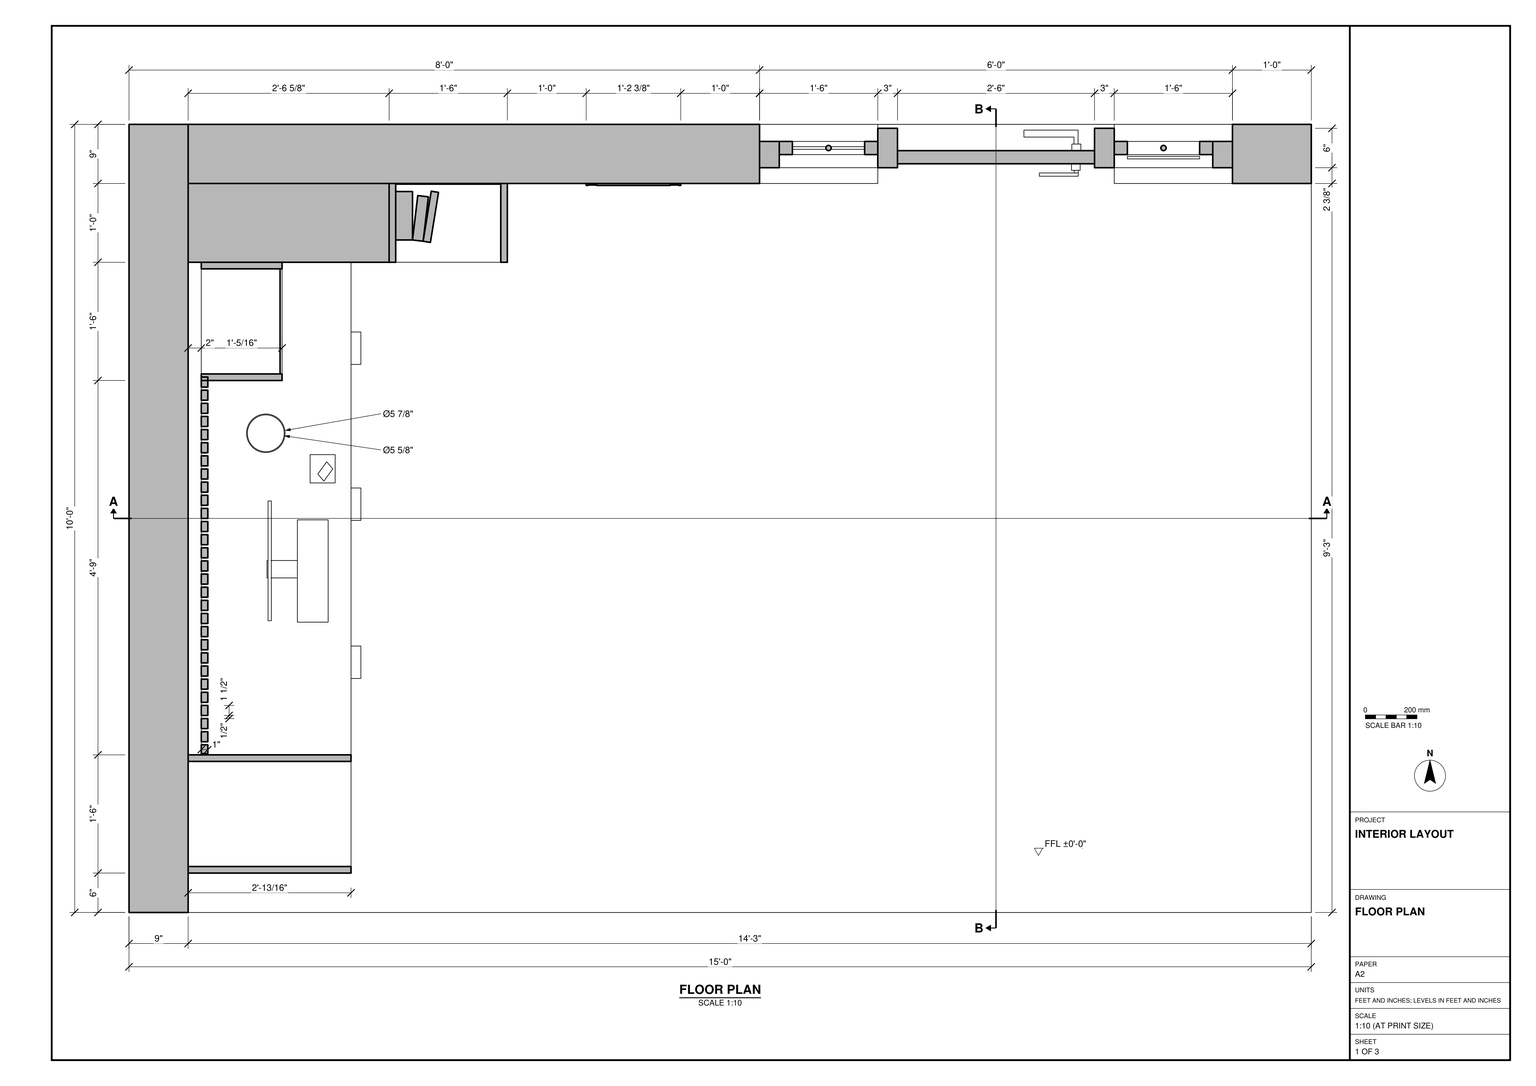
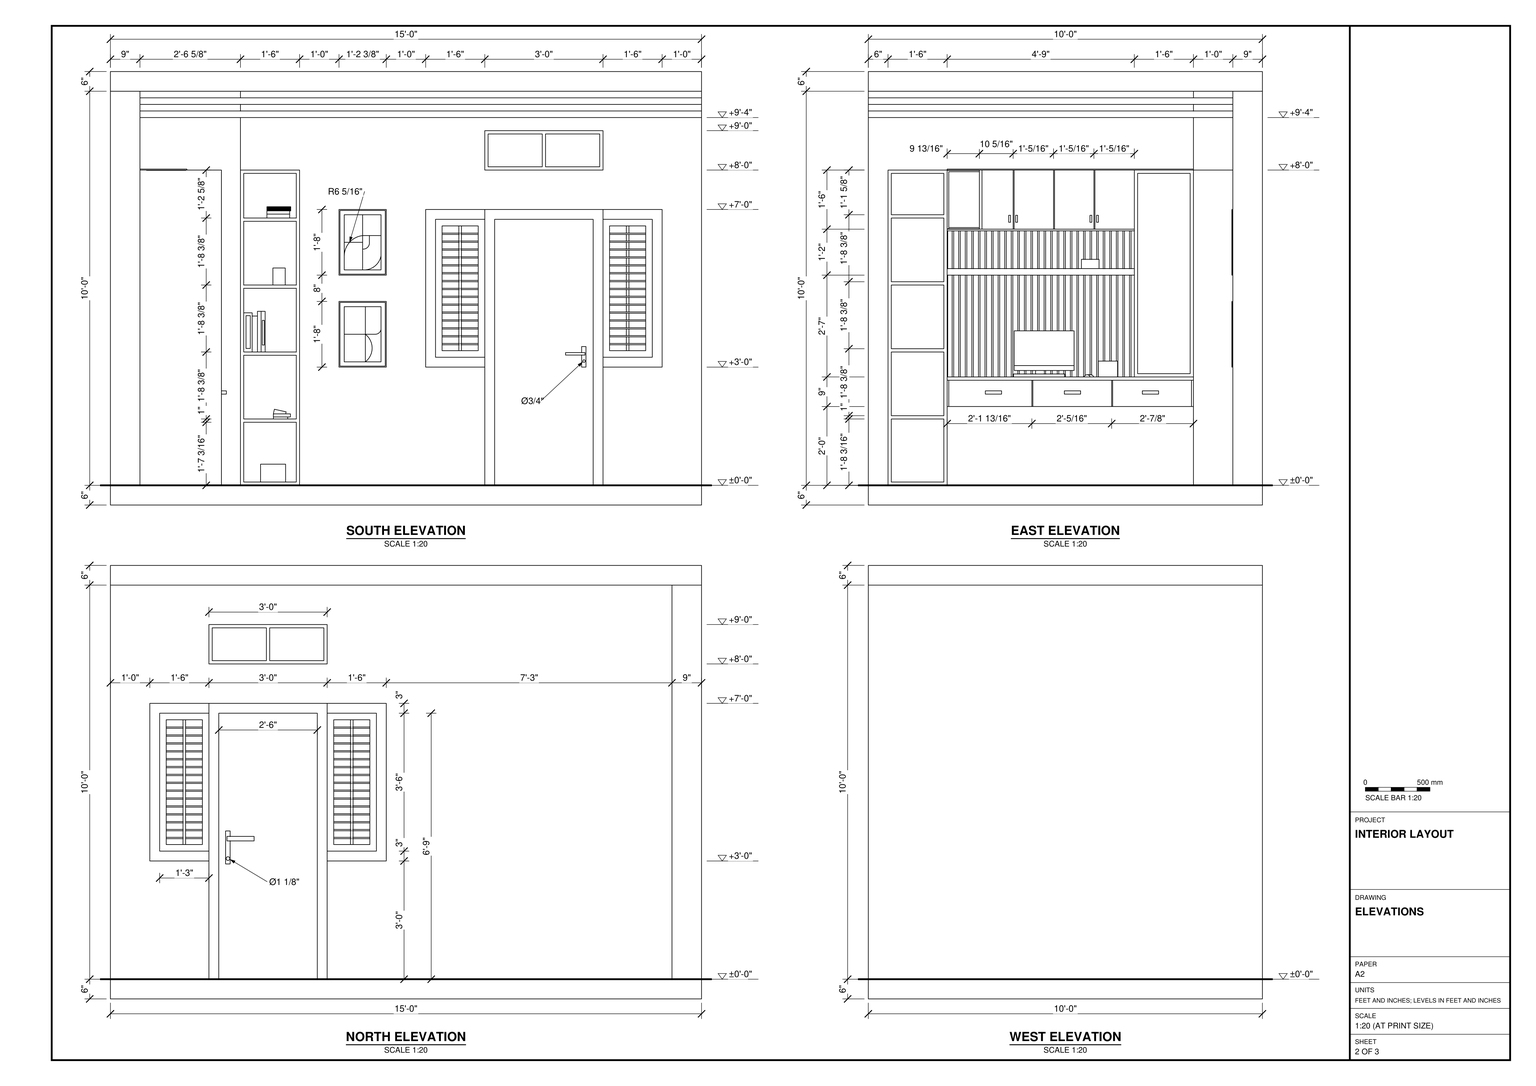
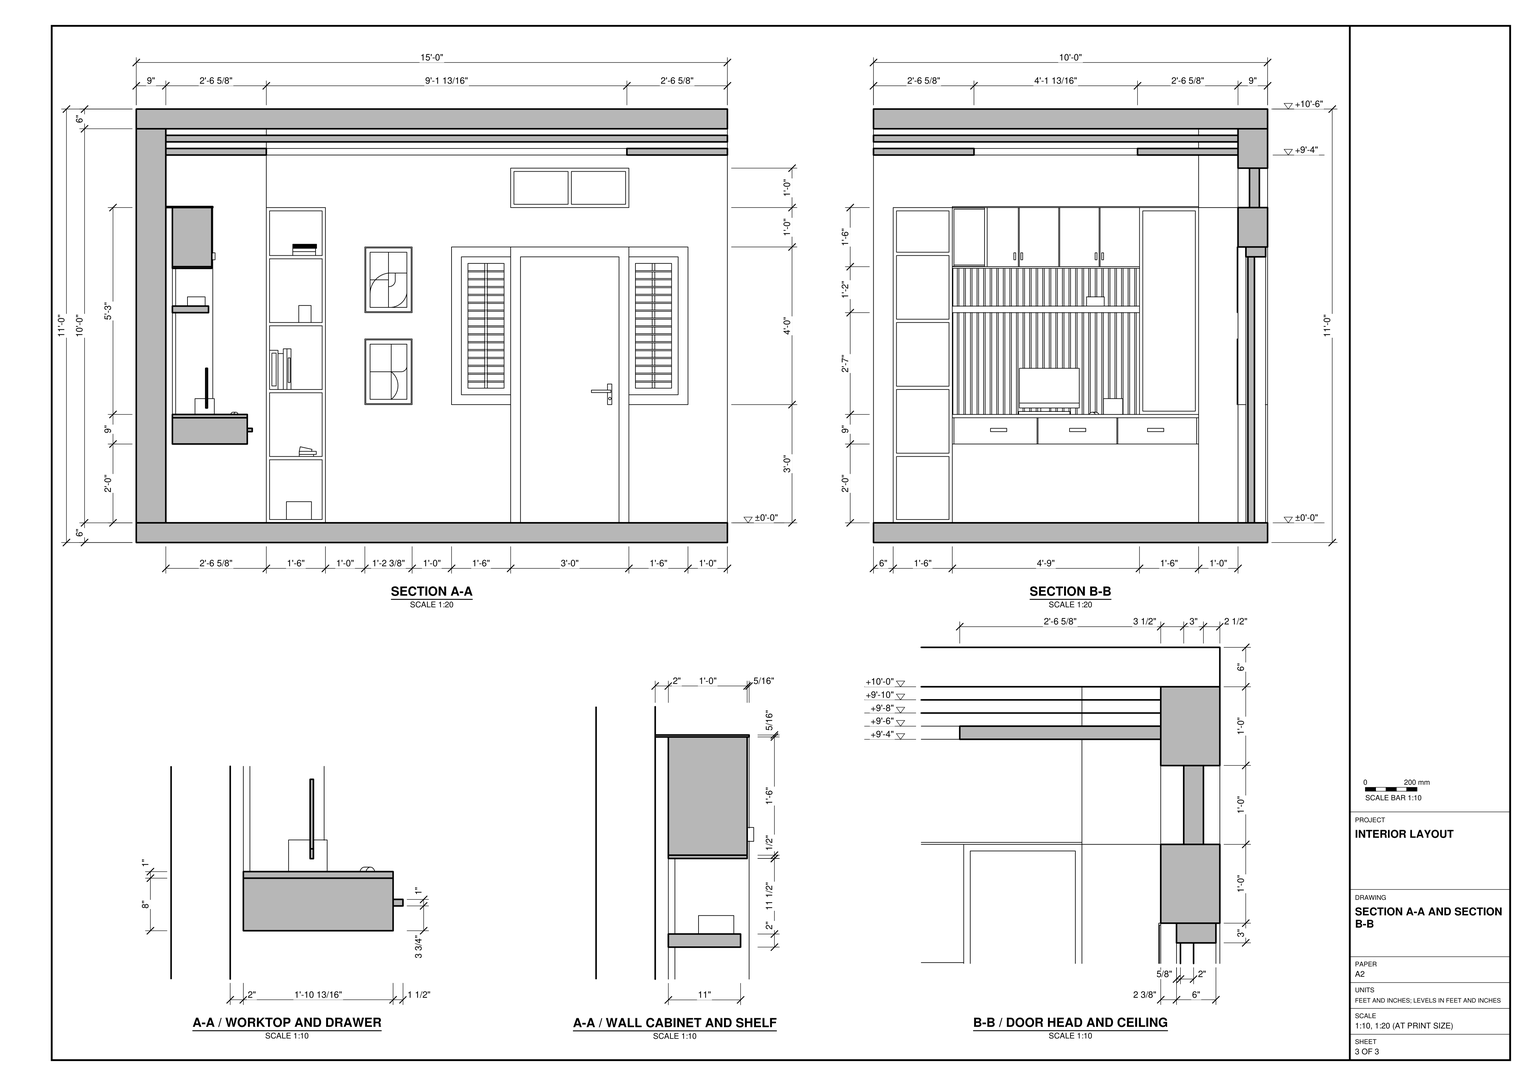
Build the interior in SketchUp from task_files/diagram_01.pdf. Work in feet and inches. Use the finished floor at ±0'-0" as the single storey datum. The model is 15'-0" along the entrance wall, 10'-0" along the workstation wall and 11'-0" high from the underside of the floor slab to the top of the roof slab.

Model the two adjoining 9" walls shown in plan, leaving the other two sides open. Include the floor and roof slabs and follow the door-head section for the stepped ceiling beneath the roof slab. Set the door toward the east end of the north wall, between two narrow louvred windows, with a separate two-pane window above it.

Fit out the west wall with the suspended worktop and drawers, vertical slatted backing, shelf, overhead cupboards and storage at each end. Use the enlarged sections to set the depths of the worktop, shelf and cupboards. Include the open shelving on the adjoining north wall, the monitor on the worktop and the pair of framed pictures between the shelving and the doorway. Decor and loose items may be any suitable library components.

Keep the walls, slabs and each furniture or joinery piece in separate groups or components, and use components for repeated parts. Save one SketchUp model as output_files/room_with_a_fitted_workstation_and_flanked_doorway.skp.

# SketchUp Ruby script. Lengths in inches.
U = 1.inch
M = Sketchup.active_model
def pt(a) = Geom::Point3d.new(a.map { |v| v * U })
def face(e, loops, mat)
  f = e.add_face(loops[0].map { |a| pt(a) })
  loops[1..].each { |l| e.add_face(l.map { |a| pt(a) }).erase! }
  f.material = f.back_material = mat if mat
  f
end
# faces: each face lists its corners as indices into pts; further lists are holes
def faces(e, pts, list, mat = nil) = list.each { |f| face(e, (f[0].is_a?(Array) ? f : [f]).map { |l| l.map { |i| pts[i] } }, mat) }
# xy, xz, yz: faces in a plane at the given z, y or x. An outline is a flat list of corners, or four numbers for a rectangle; further outlines are holes
def ring(l) = l.size == 4 ? [[l[0], l[1]], [l[2], l[1]], [l[2], l[3]], [l[0], l[3]]] : l.each_slice(2).to_a
def flat(e, list, mat, &to3) = list.each { |f| face(e, (f[0].is_a?(Array) ? f : [f]).map { |l| ring(l).map { |u, v| to3.(u, v) } }, mat) }
def xy(e, z, list, mat = nil) = flat(e, list, mat) { |x, y| [x, y, z] }
def xz(e, y, list, mat = nil) = flat(e, list, mat) { |x, z| [x, y, z] }
def yz(e, x, list, mat = nil) = flat(e, list, mat) { |y, z| [x, y, z] }
def lines(e, pts, list) = list.each { |a, b| e.add_line(pt(pts[a]), pt(pts[b])) }
# prism: a flat outline (further loops are holes) pulled along v
def prism(e, loops, v, mat = nil)
  f = face(e, loops, mat); d = Geom::Vector3d.new(v.map { |x| x * U })
  f.pushpull(f.normal.samedirection?(d) ? d.length : -d.length)
end
def box(e, o, s, mat = nil) = prism(e, [[o, [o[0] + s[0], o[1], o[2]], [o[0] + s[0], o[1] + s[1], o[2]], [o[0], o[1] + s[1], o[2]]]], [0, 0, s[2]], mat)
def at(x, y, z, deg = 0) = Geom::Transformation.translation(pt([x, y, z])) * Geom::Transformation.rotation(ORIGIN, Z_AXIS, deg.degrees)
def axes(o, x, y, z) = Geom::Transformation.new([*x, 0, *y, 0, *z, 0, *pt(o).to_a, 1])
def part(name) = M.definitions.add(name)
# library, detail: a bought-in or finely detailed component or shape, given as its bounding box
def library(name, o, s) = part(name).tap { |d| box(d.entities, o, s) }
def detail(e, o, s) = box(e.add_group.entities, o, s)
def put(e, d, t, mat = nil) = e.add_instance(d, t).tap { |i| i.material = mat if mat }
def group(e, t, mat = nil) = e.add_group.tap { |g| g.transformation = t; g.material = mat if mat }.entities
root = M.entities
M.materials.add("[0014_DarkSalmon]").color = [233, 150, 122]
M.materials.add("[0034_Wheat]").color = [245, 222, 179]
M.materials.add("[0040_Peru]").color = [205, 133, 63]
M.materials.add("[0050_LemonChiffon]").color = [255, 250, 205]
M.materials.add("[0052_FloralWhite]").color = [255, 250, 240]
M.materials.add("[0137_Black]").color = [0, 0, 0]
M.materials.add("[Color A08]").color = [102, 0, 0]
M.materials.add("[Color D02]").color = [214, 192, 128]
M.materials.add("[Color D07]").color = [153, 114, 0]
M.materials.add("[Color E01]").color = [242, 242, 193]
M.materials.add("[Color E01]1").color = [255, 255, 204]
M.materials.add("[Color L16]").color = [102, 0, 51]
M.materials.add("[Color M00]").color = [255, 255, 255]
M.materials.add("[Color M06]").color = [86, 86, 86]
M.materials.add("[Color M07]").color = [58, 58, 58]
M.materials.add("[Color M09]").color = [0, 0, 0]
M.materials.add("[Metal Aluminum Anodized]").color = [202, 209, 219]
M.materials.add("[Translucent Glass Blue]").color = [107, 160, 255]
M.materials.add("[Translucent Glass Gray]").color = [128, 128, 128]
M.materials.add("[Vegetation Juniper]").color = [99, 128, 70]
M.materials.add("[Wood Veneer 01]").color = [112, 65, 34]
M.materials.add("[Wood Veneer 01]1").color = [84, 49, 25]
c1 = part("Group\#11")
prism(c1.entities,[[[0,0.27,0.01],[0,0.22,0],[0,0.17,0],[0,0.12,0.02],[0,0.07,0.04],[0,0.04,0.08],[0,0.01,0.13],[0,0,0.18],[0,0,0.23],[0,0.02,0.28],[0,0.04,0.33],[0,0.08,0.36],[0,0.13,0.39],[0,0.18,0.4],[0,0.23,0.4],[0,0.28,0.38],[0,0.33,0.35],[0,0.36,0.32],[0,0.39,0.27],[0,0.4,0.22],[0,0.4,0.17],[0,0.38,0.12],[0,0.35,0.07],[0,0.32,0.04]]],[11,0,0])
c2 = part("Group\#9")
xy(c2.entities,0,[[0,0,15,2]])
xy(c2.entities,2,[[[2,0,13,2],[7.5,0.6,7.4,0.61,7.3,0.65,7.22,0.72,7.15,0.8,7.11,0.9,7.1,1,7.11,1.1,7.15,1.2,7.22,1.28,7.3,1.35,7.4,1.39,7.5,1.4,7.6,1.39,7.7,1.35,7.78,1.28,7.85,1.2,7.89,1.1,7.9,1,7.89,0.9,7.85,0.8,7.78,0.72,7.7,0.65,7.6,0.61]]])
xy(c2.entities,40,[[[2,0,13,2],[7.5,0.6,7.6,0.61,7.7,0.65,7.78,0.72,7.85,0.8,7.89,0.9,7.9,1,7.89,1.1,7.85,1.2,7.78,1.28,7.7,1.35,7.6,1.39,7.5,1.4,7.4,1.39,7.3,1.35,7.22,1.28,7.15,1.2,7.11,1.1,7.1,1,7.11,0.9,7.15,0.8,7.22,0.72,7.3,0.65,7.4,0.61]]])
xy(c2.entities,42,[[0,0,15,2]])
xz(c2.entities,0,[[[0,0,15,42],[2,2,13,40]]])
xz(c2.entities,2,[[[0,0,15,42],[2,2,13,40]]])
yz(c2.entities,0,[[0,0,2,42]])
yz(c2.entities,2,[[0,2,2,40]])
yz(c2.entities,13,[[0,2,2,40]])
yz(c2.entities,15,[[0,0,2,42]])
p = [[7.3,0.65,2],[7.4,0.61,2],[7.4,0.61,40],[7.3,0.65,40],[7.5,0.6,2],[7.5,0.6,40],
  [7.6,0.61,2],[7.6,0.61,40],[7.7,0.65,2],[7.7,0.65,40],[7.15,0.8,2],[7.22,0.72,2],
  [7.22,0.72,40],[7.15,0.8,40],[7.78,0.72,2],[7.78,0.72,40],[7.85,0.8,2],[7.85,0.8,40],
  [7.11,0.9,2],[7.11,0.9,40],[7.89,0.9,2],[7.89,0.9,40],[7.1,1,2],[7.1,1,40],
  [7.9,1,2],[7.9,1,40],[7.11,1.1,2],[7.11,1.1,40],[7.89,1.1,2],[7.89,1.1,40],
  [7.15,1.2,2],[7.15,1.2,40],[7.85,1.2,2],[7.85,1.2,40],[7.22,1.28,2],[7.22,1.28,40],
  [7.78,1.28,2],[7.78,1.28,40],[7.3,1.35,2],[7.3,1.35,40],[7.4,1.39,2],[7.4,1.39,40],
  [7.7,1.35,2],[7.6,1.39,2],[7.6,1.39,40],[7.7,1.35,40],[7.5,1.4,2],[7.5,1.4,40]]
faces(c2.entities,p,[[0,1,2,3],[1,4,5,2],[4,6,7,5],[6,8,9,7],[10,11,12,13],[11,0,3,12],[8,14,15,9],[14,16,17,15],
  [18,10,13,19],[16,20,21,17],[22,18,19,23],[20,24,25,21],[26,22,23,27],[24,28,29,25],[30,26,27,31],[28,32,33,29],
  [34,30,31,35],[32,36,37,33],[38,34,35,39],[40,38,39,41],[42,43,44,45],[36,42,45,37],[46,40,41,47],[43,46,47,44]])
c3 = part("Group\#28")
box(c3.entities,[0,0,0],[1,1.53,44.5])
c4 = part("Group\#30")
box(c4.entities,[0,0,0],[1,0.5625,2.125])
c5 = part("Group\#31")
box(c5.entities,[0,0,0],[1.5,4.9375,1])
c6 = library("Group\#43",[0,0,0],[171,111,2])
c7 = library("Group\#45",[0,0,0],[7.625,7.62,5.4375])
c8 = library("Group\#50",[0,0,0],[5.875,5.87,4.8125])
box(root,[40.6,110.9,7],[16,0.1,94],"[Color E01]")
xz(root,114.5,[[115,103,131.5,113],[132.5,103,149,113]],"[Translucent Glass Blue]")
yz(root,23,[[82,40,98,101],[24.5,84.5,33.8125,101.5]],"[Translucent Glass Gray]")
# 5 loose lines left out
g1 = group(root,at(9,111,6),"[0050_LemonChiffon]")
prism(g1,[[[105,9,0],[0,9,0],[0,9,120],[171,9,120],[171,9,0],[141,9,0],[141,9,36],[159,9,36],[159,9,84],[141,9,84],[105,9,84],[87,9,84],[87,9,36],[105,9,36]],[[105,9,108],[105,9,96],[141,9,96],[141,9,108]]],[0,-9,0])
g2 = group(root,at(96,112.1,6),"[Wood Veneer 01]")
g3 = group(g2,at(42.59,0,36),"[Metal Aluminum Anodized]")
box(g3,[0,0,3.67],[5.92,0.5,0.75])
g4 = group(g3,at(4.9,0.5,0))
xy(g4,0,[[0,0.4,1.32,1.4]])
xy(g4,3.86,[[0.41,0,1.02,0.4]])
xy(g4,4.42,[[0.41,0,1.02,0.4]])
xy(g4,6.26,[[0,0.4,1.32,1.4]])
xz(g4,0,[[0.41,3.86,1.02,4.42]])
xz(g4,0.4,[[[0,0,1.32,6.26],[0.72,1.47,0.625,1.49,0.53,1.52,0.46,1.58,0.4,1.66,0.36,1.75,0.35,1.85,0.36,1.94,0.4,2.04,0.46,2.11,0.53,2.17,0.625,2.21,0.72,2.22,0.82,2.21,0.91,2.17,0.99,2.11,1.05,2.04,1.08,1.94,1.1,1.85,1.08,1.75,1.05,1.66,0.99,1.58,0.91,1.52,0.82,1.49],[0.41,3.86,1.02,4.42]]])
xz(g4,1.4,[[0,0,1.32,6.26]])
xz(g4,1.84,[[0.72,1.47,0.82,1.49,0.91,1.52,0.99,1.58,1.05,1.66,1.08,1.75,1.1,1.85,1.08,1.94,1.05,2.04,0.99,2.11,0.91,2.17,0.82,2.21,0.72,2.22,0.625,2.21,0.53,2.17,0.46,2.11,0.4,2.04,0.36,1.94,0.35,1.85,0.36,1.75,0.4,1.66,0.46,1.58,0.53,1.52,0.625,1.49]])
yz(g4,0,[[0.4,0,1.4,6.26]])
yz(g4,0.41,[[0,3.86,0.4,4.42]])
yz(g4,1.02,[[0,3.86,0.4,4.42]])
yz(g4,1.32,[[0.4,0,1.4,6.26]])
p = [[0.46,0.4,1.58],[0.53,0.4,1.52],[0.53,1.84,1.52],[0.46,1.84,1.58],[0.625,0.4,1.49],[0.625,1.84,1.49],
  [0.72,0.4,1.47],[0.72,1.84,1.47],[0.82,0.4,1.49],[0.82,1.84,1.49],[0.91,0.4,1.52],[0.91,1.84,1.52],
  [0.99,0.4,1.58],[0.99,1.84,1.58],[0.4,0.4,1.66],[0.4,1.84,1.66],[1.05,0.4,1.66],[1.05,1.84,1.66],
  [0.36,0.4,1.75],[0.36,1.84,1.75],[1.08,0.4,1.75],[1.08,1.84,1.75],[0.35,0.4,1.85],[0.35,1.84,1.85],
  [0.36,0.4,1.94],[0.36,1.84,1.94],[1.1,0.4,1.85],[1.08,0.4,1.94],[1.08,1.84,1.94],[1.1,1.84,1.85],
  [0.4,0.4,2.04],[0.4,1.84,2.04],[1.05,0.4,2.04],[1.05,1.84,2.04],[0.46,0.4,2.11],[0.46,1.84,2.11],
  [0.99,0.4,2.11],[0.99,1.84,2.11],[0.53,0.4,2.17],[0.53,1.84,2.17],[0.91,0.4,2.17],[0.91,1.84,2.17],
  [0.625,0.4,2.21],[0.625,1.84,2.21],[0.72,0.4,2.22],[0.72,1.84,2.22],[0.82,0.4,2.21],[0.82,1.84,2.21]]
faces(g4,p,[[0,1,2,3],[1,4,5,2],[4,6,7,5],[6,8,9,7],[8,10,11,9],[10,12,13,11],[14,0,3,15],[12,16,17,13],
  [18,14,15,19],[16,20,21,17],[22,18,19,23],[24,22,23,25],[26,27,28,29],[20,26,29,21],[30,24,25,31],[27,32,33,28],
  [34,30,31,35],[32,36,37,33],[38,34,35,39],[36,40,41,37],[42,38,39,43],[44,42,43,45],[46,44,45,47],[40,46,47,41]])
g5 = group(g2,at(18,1.3,0))
prism(g5,[[[36,6,0],[33,6,0],[33,6,81],[3,6,81],[3,6,0],[0,6,0],[0,6,84],[36,6,84]]],[0,-6,0])
g6 = group(g2,at(54,1.3,36))
prism(g6,[[[15,4,45],[0,4,45],[0,4,48],[18,4,48],[18,4,0],[0,4,0],[0,4,3],[15,4,3]]],[0,-4,0])
# 1 loose lines left out
g7 = group(g2,at(0,1.3,36))
prism(g7,[[[18,4,48],[18,4,45],[3,4,45],[3,4,3],[18,4,3],[18,4,0],[0,4,0],[0,4,48]]],[0,-4,0])
# 1 loose lines left out
g8 = group(g2,at(21,1.9,0))
box(g8,[0,0,0],[30,2,81])
g9 = group(g2,at(54,1.84,39))
put(g9,c1,at(2,0.8,13.4))
put(g9,c1,at(2,0.8,3.8))
put(g9,c1,at(2,0.8,8.6))
put(g9,c1,at(2,0.8,20.6))
put(g9,c1,at(2,0.8,11))
put(g9,c1,at(2,0.8,15.8))
put(g9,c1,at(2,0.8,25.4))
put(g9,c1,at(2,0.8,23))
put(g9,c2,at(0,1.46,0))
put(g9,c1,at(2,0.8,18.2))
put(g9,c1,at(2,0.8,6.2))
put(g9,c1,at(2,0.8,37.4))
put(g9,c1,at(2,0.8,32.6))
put(g9,c1,at(2,0.8,35))
put(g9,c1,at(2,0.8,30.2))
put(g9,c1,at(2,0.8,27.8))
g10 = group(g2,at(3,3.3,39))
put(g10,c1,at(2,0.8,13.4))
put(g10,c1,at(2,0.8,3.8))
put(g10,c1,at(2,0.8,8.6))
put(g10,c1,at(2,0.8,20.6))
put(g10,c1,at(2,0.8,11))
put(g10,c1,at(2,0.8,15.8))
put(g10,c1,at(2,0.8,25.4))
put(g10,c1,at(2,0.8,23))
put(g10,c2,at(0,0,0))
put(g10,c1,at(2,0.8,18.2))
put(g10,c1,at(2,0.8,6.2))
put(g10,c1,at(2,0.8,37.4))
put(g10,c1,at(2,0.8,32.6))
put(g10,c1,at(2,0.8,35))
put(g10,c1,at(2,0.8,30.2))
put(g10,c1,at(2,0.8,27.8))
g11 = group(root,at(114,115.5,102))
prism(g11,[[[0,-1,12],[0,-1,0],[36,-1,0],[36,-1,12]],[[17.5,-1,11],[17.5,-1,1],[1,-1,1],[1,-1,11]],[[18.5,-1,11],[35,-1,11],[35,-1,1],[18.5,-1,1]]],[0,3,0])
g12 = group(root,at(0,0,6),"[0050_LemonChiffon]")
box(g12,[0,0,0],[9,120,120])
g13 = group(root,at(9,99,6),"[0050_LemonChiffon]")
xy(g13,0,[[0,0,30.6,12]])
xy(g13,120,[[0,0,30.6,12]])
xz(g13,0,[[0,0,30.6,112],[0,112,30.6,120]])
xz(g13,12,[[0,0,30.6,120]])
yz(g13,0,[[0,0,12,120]])
yz(g13,30.6,[[0,0,12,112],[0,112,12,120]])
g14 = group(root,at(0,0,0))
box(g14,[0,0,0],[180,120,6])
g15 = group(root,at(9,24,30))
g16 = group(g15,at(2,57,9),"[Wood Veneer 01]1")
xy(g16,0,[[0,0,12.3,18]])
xy(g16,1,[[0,1,12.3,17]])
xy(g16,62,[[0,1,12.3,17]])
xy(g16,63,[[0,0,12.3,18]])
xz(g16,0,[[0,0,12.3,63]])
xz(g16,1,[[0,1,12.3,62]])
xz(g16,17,[[0,1,12.3,62]])
xz(g16,18,[[0,0,12.3,63]])
yz(g16,0,[[[0,0,18,63],[1,1,17,62]]])
yz(g16,12.3,[[[0,0,18,63],[1,1,17,62]]],"[Color M00]")
g17 = group(g15,at(2,0,8),"[Wood Veneer 01]1")
box(g17,[0,0,0],[22.8,75,1])
g18 = group(g15,at(2,0,54))
xy(g18,0,[[0,0,12,9.8125],[0,9.8125,12,10.61],[0,10.61,12,20.1],[0,20.1,11.7,20.4],[0,20.4,12,32.4],
  [0,32.4,12,32.7],[0,32.7,12,44.7],[0,44.7,11.7,45],[0,45,12,57]],"[Color M00]")
xy(g18,17.9,[[0,0,12,9.8125]],"[Color M00]")
xy(g18,18,[[0,9.8125,12,10.61],[0,10.61,12,20.1],[0,20.1,11.7,20.4],[0,20.4,12,32.4],[0,32.4,12,32.7],
  [0,32.7,12,44.7],[0,44.7,11.7,45],[0,45,12,57]],"[Color M00]")
xz(g18,0,[[0,0,12,17.9]],"[Color M00]")
xz(g18,9.8125,[[0,0,12,17.9],[0,17.9,12,18]],"[Color M00]")
xz(g18,10.61,[[0,0,12,18]],"[Color M00]")
xz(g18,20.1,[[0,0,11.7,18],[11.7,0,12,18]],"[Color M00]")
xz(g18,20.4,[[0,0,11.7,18],[11.7,0,12,18]],"[Color M00]")
xz(g18,32.4,[[0,0,12,18]],"[Color M00]")
xz(g18,32.7,[[0,0,12,18]],"[Color M00]")
xz(g18,44.7,[[0,0,11.7,18],[11.7,0,12,18]],"[Color M00]")
xz(g18,45,[[0,0,11.7,18],[11.7,0,12,18]],"[Color M00]")
xz(g18,57,[[0,0,12,18]],"[Color M00]")
yz(g18,0,[[9.8125,0,10.61,18],[10.61,0,20.1,18],[20.1,0,20.4,18],[20.4,0,32.4,18],[32.4,0,32.7,18],
  [32.7,0,44.7,18],[44.7,0,45,18],[45,0,57,18],[0,17.9,9.8125,18]],"[Color M00]")
yz(g18,11.7,[[20.1,0,20.4,18],[44.7,0,45,18]],"[Color M00]")
yz(g18,12,[[0,0,9.8125,0,9.8125,0.5,0.5,0.5,0.5,17.5,9.8125,17.5,9.8125,17.9,0,17.9],[9.8125,0,10.61,18],[10.61,0,20.1,18],[20.4,0,32.4,18],[32.4,0,32.7,18],
  [32.7,0,44.7,18],[45,0,57,18]],"[Color M00]")
g19 = group(g15,at(2,-1,40),"[Wood Veneer 01]1")
box(g19,[0,1,0],[11,57,2])
g20 = group(g15,at(2,0,0))
xy(g20,0,[[0,0,22.8,0.5],[0,0.5,22.8,25.8],[0,25.8,22.5,26.1],[0,26.1,22.8,50.1],[0,50.1,22.5,50.4],
  [0,50.4,22.8,74.4],[0,74.4,22.8,75]])
xy(g20,8,[[0,0,22.8,0.5],[0,0.5,22.8,25.8],[0,25.8,22.5,26.1],[22.5,25.8,22.8,26.1],[0,26.1,22.8,50.1],
  [0,50.1,22.5,50.4],[22.5,50.1,22.8,50.4],[0,50.4,22.8,74.4],[0,74.4,22.8,75]])
xz(g20,0,[[0,0,22.8,8]])
xz(g20,0.5,[[0,0,22.8,8]])
xz(g20,25.8,[[0,0,22.5,8],[22.5,0,22.8,8]])
xz(g20,26.1,[[0,0,22.5,8],[22.5,0,22.8,8]])
xz(g20,50.1,[[0,0,22.5,8],[22.5,0,22.8,8]])
xz(g20,50.4,[[0,0,22.5,8],[22.5,0,22.8,8]])
xz(g20,74.4,[[0,0,22.8,8]])
xz(g20,75,[[0,0,22.8,8]])
yz(g20,0,[[0,0,0.5,8],[0.5,0,25.8,8],[25.8,0,26.1,8],[26.1,0,50.1,8],[50.1,0,50.4,8],
  [50.4,0,74.4,8],[74.4,0,75,8]])
yz(g20,22.5,[[25.8,0,26.1,8],[50.1,0,50.4,8]])
yz(g20,22.8,[[0,0,0.5,8],[0.5,0,25.8,8],[26.1,0,50.1,8],[50.4,0,74.4,8],[74.4,0,75,8]])
g21 = group(root,at(39.6,99,6),"[Wood Veneer 01]1")
prism(g21,[[[0,12,0],[0,12,96],[18,12,96],[18,12,0]],[[1,12,61],[17,12,61],[17,12,80.4],[1,12,80.4]],[[1,12,40.6],[17,12,40.6],[17,12,60],[1,12,60]],[[1,12,39.6],[1,12,20.2],[17,12,20.2],[17,12,39.6]],[[17,12,19.2],[1,12,19.2],[1,12,1],[17,12,1]],[[1,12,95],[1,12,81.4],[17,12,81.4],[17,12,95]]],[0,-12,0])
g22 = group(root,at(11,24,83.5),"[Wood Veneer 01]1")
box(g22,[0,0,0],[12,57,0.5])
g23 = group(root,at(11,24,39),"[Color D02]")
put(g23,c3,at(0,4,0))
g24 = group(g23,at(0,0,0))
box(g24,[0,0.1875,0],[1,1.34,44.5])
put(g23,c3,at(0,2,0))
put(g23,c3,at(0,6,0))
put(g23,c3,at(0,56,0))
put(g23,c3,at(0,46,0))
put(g23,c3,at(0,44,0))
put(g23,c3,at(0,50,0))
put(g23,c3,at(0,54,0))
put(g23,c3,at(0,52,0))
put(g23,c3,at(0,48,0))
put(g23,c3,at(0,20,0))
put(g23,c3,at(0,34,0))
put(g23,c3,at(0,38,0))
put(g23,c3,at(0,40,0))
put(g23,c3,at(0,36,0))
put(g23,c3,at(0,18,0))
put(g23,c3,at(0,8,0))
put(g23,c3,at(0,14,0))
put(g23,c3,at(0,22,0))
put(g23,c3,at(0,26,0))
put(g23,c3,at(0,30,0))
put(g23,c3,at(0,12,0))
put(g23,c3,at(0,10,0))
put(g23,c3,at(0,24,0))
put(g23,c3,at(0,28,0))
put(g23,c3,at(0,16,0))
put(g23,c3,at(0,32,0))
put(g23,c3,at(0,42,0))
g25 = group(root,at(9,24,102),"[Wood Veneer 01]1")
box(g25,[0,0,0],[14.3,75,0.3])
put(root,c4,at(23,69.49,86.1),"[Wood Veneer 01]1")
put(root,c4,at(23,67.49,86.1),"[Wood Veneer 01]1")
put(root,c4,at(23,44.86,86.1),"[Wood Veneer 01]1")
put(root,c4,at(23,42.74,86.1),"[Wood Veneer 01]1")
put(root,c5,at(33.8,35.63,33.77),"[Wood Veneer 01]1")
put(root,c5,at(33.8,59.7,33.77),"[Wood Veneer 01]1")
put(root,c5,at(33.8,83.45,33.77),"[Wood Veneer 01]1")
g26 = group(root,at(21,44.2,39))
box(g26,[4.625,0,0],[4.6875,15.58,0.91])
g27 = group(g26,at(0.17,0.22,1.97))
xy(g27,0,[[0,0,0.5,18.23]])
xy(g27,1.49,[[0,0,0.5,18.23]])
xy(g27,12.08,[[0,0,0.5,18.23]])
xz(g27,0,[[0,0,0.5,1.49],[0,1.49,0.5,12.08]])
xz(g27,18.23,[[0,0,0.5,1.49],[0,1.49,0.5,12.08]])
yz(g27,0,[[0,0,18.23,1.49],[0,1.49,18.23,12.08]])
yz(g27,0.5,[[0,0,18.23,1.49]])
yz(g27,0.5,[[0,1.49,18.23,12.08]],"[Color M09]")
g28 = group(g26,at(0,6.74,0))
prism(g28,[[[0,0,0],[4.625,0,0],[4.625,0,0.29],[0.17,0,0.29],[0.17,0,2.78],[0,0,2.78]]],[0,2.65,0])
g29 = group(root,at(47.66,99.78,87.4))
box(g29,[0,0,0],[6.9375,9.75,1.1875])
g30 = group(root,at(47.66,101.36,88.59))
box(g30,[0,0,0],[6.9375,6.1,1])
g31 = group(root,at(47.66,99.8,89.59))
xy(g31,0,[[0,-0.125,7.25,7.67]])
xy(g31,0.08,[[0.2,-0.125,7.25,0.1]])
xy(g31,0.16,[[0.2,-0.125,7.25,0.1]])
xy(g31,0.23,[[0.2,-0.125,7.25,-0.1]])
xy(g31,0.31,[[0.2,-0.125,7.25,-0.1]])
xy(g31,0.38,[[0.2,-0.125,7.25,-0.1]])
xy(g31,0.46,[[0.2,-0.125,7.25,-0.1]])
xy(g31,0.53,[[0.2,-0.125,7.25,-0.1]])
xy(g31,0.61,[[0.2,-0.125,7.25,-0.1]])
xy(g31,0.68,[[0.2,-0.125,7.25,-0.1]])
xy(g31,0.76,[[0.2,-0.125,7.25,-0.1]])
xy(g31,0.83,[[0.2,-0.125,7.25,-0.1]])
xy(g31,0.91,[[0.2,-0.125,7.25,-0.1]])
xy(g31,0.98,[[0.2,-0.125,7.25,-0.1]])
xy(g31,1.06,[[0.2,-0.125,7.25,-0.1]])
xy(g31,1.13,[[0.2,-0.125,7.25,-0.1]])
xy(g31,1.21,[[0.2,-0.125,7.25,-0.1]])
xy(g31,1.25,[[0,-0.125,7.25,7.67]])
xz(g31,-0.125,[[0,0,7.25,0,7.25,0.08,0.2,0.08,0.2,0.16,7.25,0.16,7.25,0.23,0.2,0.23,0.2,0.31,7.25,0.31,7.25,0.38,0.2,0.38,0.2,0.46,7.25,0.46,7.25,0.53,0.2,0.53,0.2,0.61,7.25,0.61,7.25,0.68,0.2,0.68,0.2,0.76,7.25,0.76,7.25,0.83,0.2,0.83,0.2,0.91,7.25,0.91,7.25,0.98,0.2,0.98,0.2,1.06,7.25,1.06,7.25,1.13,0.2,1.13,0.2,1.21,7.25,1.21,7.25,1.25,0,1.25]])
xz(g31,-0.1,[[0.2,0.23,7.25,0.31],[0.2,0.38,7.25,0.46],[0.2,0.53,7.25,0.61],[0.2,0.68,7.25,0.76],[0.2,0.83,7.25,0.91],
  [0.2,0.98,7.25,1.06],[0.2,1.13,7.25,1.21]])
xz(g31,0.1,[[0.2,0.08,7.25,0.16]])
xz(g31,7.67,[[0,0,7.25,1.25]])
yz(g31,0,[[-0.125,0,7.67,1.25]])
yz(g31,0.2,[[-0.125,0.08,0.1,0.16],[-0.125,0.23,-0.1,0.31],[-0.125,0.38,-0.1,0.46],[-0.125,0.53,-0.1,0.61],[-0.125,0.68,-0.1,0.76],
  [-0.125,0.83,-0.1,0.91],[-0.125,0.98,-0.1,1.06],[-0.125,1.13,-0.1,1.21]])
yz(g31,7.25,[[-0.125,0,7.67,0,7.67,1.25,-0.125,1.25,-0.125,1.21,-0.1,1.21,-0.1,1.13,-0.125,1.13,-0.125,1.06,-0.1,1.06,-0.1,0.98,-0.125,0.98,-0.125,0.91,-0.1,0.91,-0.1,0.83,-0.125,0.83,-0.125,0.76,-0.1,0.76,-0.1,0.68,-0.125,0.68,-0.125,0.61,-0.1,0.61,-0.1,0.53,-0.125,0.53,-0.125,0.46,-0.1,0.46,-0.1,0.38,-0.125,0.38,-0.125,0.31,-0.1,0.31,-0.1,0.23,-0.125,0.23,-0.125,0.16,0.1,0.16,0.1,0.08,-0.125,0.08]])
g32 = group(root,at(40.6,102.03,46.6),"[Color M09]")
xy(g32,0,[[5.29,0,4.18,0.18,5.41,7.8,6.52,7.62],[4.18,0.18,2.5625,0.37,3.36,7.13,4.97,6.94],[0,0.37,2.5625,7.74]],"[Color M00]")
xy(g32,10.95,[[4.18,0.18,4.97,6.94,3.36,7.13,2.5625,0.37]],"[Color M00]")
xy(g32,11.9375,[[0,0.37,2.5625,7.74]],"[Color M00]")
xy(g32,12.39,[[5.29,0,6.52,7.62,5.41,7.8,4.18,0.18]],"[Color M00]")
xz(g32,0.37,[[[0,0,2.5625,11.9375],[0.69,1.07,2,11.07]]],"[Color M00]")
xz(g32,0.37,[[0.69,1.07,2,11.07]],"[Color M07]")
xz(g32,7.74,[[0,0,2.5625,11.9375]],"[Color M00]")
yz(g32,0,[[0.37,0,7.74,11.9375]],"[Color M00]")
yz(g32,2.5625,[[0.37,0,7.74,11.9375]],"[Color M00]")
p = [[4.18,0.18,10.95],[4.18,0.18,0],[5.29,0,0],[5.29,0,12.39],[4.18,0.18,12.39],[6.52,7.62,0],
  [6.52,7.62,12.39],[6.26,6.01,9.625],[6.26,6.01,2.125],[5.66,2.31,2.125],[5.66,2.31,9.625],[2.5625,0.37,10.95],
  [2.5625,0.37,0],[4.97,6.94,0],[4.97,6.94,10.95],[5.41,7.8,0],[5.41,7.8,12.39],[3.36,7.13,0],
  [3.36,7.13,10.95]]
faces(g32,p,[[0,1,2,3,4],[[2,5,6,3],[7,8,9,10]],[1,13,14,0],[15,1,0,4,16],[17,12,11,18],[17,18,14,13],[15,16,6,5]],"[Color M00]")
faces(g32,p,[[11,12,1,0]],"[Color M06]")
faces(g32,p,[[8,7,10,9]],"[Color L16]")
g33 = group(root,at(69.6,110.7,70))
xy(g33,0,[[0,0,14.4,0.3]])
xy(g33,0.3,[[0.3,0,14.1,0.1],[0.3,0.1,14.1,0.3]])
xy(g33,1.6,[[1.6,0,12.8,0.1]])
xy(g33,18.4,[[1.6,0,12.8,0.1]])
xy(g33,19.7,[[0.3,0,14.1,0.1],[0.3,0.1,14.1,0.3]])
xy(g33,20,[[0,0,14.4,0.3]])
xz(g33,0,[[7.2,1.6,7.2,7.94,7.48,7.93,7.75,7.97,8.02,8.04,8.27,8.15,8.51,8.3,8.72,8.48,8.9,8.69,9.05,8.93,9.16,9.18,9.23,9.45,9.27,9.72,9.26,10,9.26,12.06,12.8,12.06,12.8,5.93,12.71,5.48,12.44,4.72,12.06,4.01,11.5625,3.36,10.98,2.8,10.32,2.33,9.59,1.97,8.8125,1.72,8.02,1.6],[1.6,10,1.6,18.4,7.2,18.4,7.2,12.06,6.45,11.93,5.71,11.71,5.01,11.4,4.35,11.01,3.75,10.54,3.21,10]],"[0014_DarkSalmon]")
xz(g33,0,[[8.02,1.6,8.8125,1.72,9.59,1.97,10.32,2.33,10.98,2.8,11.5625,3.36,12.06,4.01,12.44,4.72,12.71,5.48,12.8,5.93,12.8,1.6],[1.6,5.8,1.6,10,3.21,10,3.2,10,2.73,9.4,2.33,8.74,2.01,8.05,1.79,7.32,1.65,6.5625],[7.2,12.06,12.8,18.4]],"[0034_Wheat]")
xz(g33,0,[[7.48,7.93,7.2,7.94,7.2,12.06,9.26,12.06,9.26,10,9.27,9.72,9.23,9.45,9.16,9.18,9.05,8.93,8.9,8.69,8.72,8.48,8.51,8.3,8.27,8.15,8.02,8.04,7.75,7.97]],"[0040_Peru]")
xz(g33,0,[[[0,0,14.4,20],[0.3,0.3,14.1,19.7]],[1.6,1.6,1.6,5.8,1.65,6.5625,1.79,7.32,2.01,8.05,2.33,8.74,2.73,9.4,3.2,10,7.2,10,7.2,1.6],[3.21,10,3.75,10.54,4.35,11.01,5.01,11.4,5.71,11.71,6.45,11.93,7.2,12.06,7.2,10]],"[Color M09]")
xz(g33,0.1,[[[0.3,0.3,14.1,19.7],[1.6,1.6,12.8,18.4]]],"[Color M00]")
xz(g33,0.3,[[[0,0,14.4,20],[0.3,0.3,14.1,19.7]]])
yz(g33,0,[[0,0,0.3,20]])
yz(g33,0.3,[[0,0.3,0.1,19.7],[0.1,0.3,0.3,19.7]])
yz(g33,1.6,[[0,1.6,0.1,18.4]])
yz(g33,12.8,[[0,1.6,0.1,18.4]])
yz(g33,14.1,[[0,0.3,0.1,19.7],[0.1,0.3,0.3,19.7]])
yz(g33,14.4,[[0,0,0.3,20]])
g34 = group(root,at(69.6,110.7,42),"[0034_Wheat]")
xy(g34,0,[[0,0,14.4,0.3]],"[Color E01]1")
xy(g34,0.3,[[0.3,0,14.1,0.1],[0.3,0.1,14.1,0.3]],"[Color E01]1")
xy(g34,1.6,[[1.6,0,12.8,0.1]],"[Color E01]1")
xy(g34,18.4,[[1.6,0,12.8,0.1]],"[Color E01]1")
xy(g34,19.7,[[0.3,0,14.1,0.1],[0.3,0.1,14.1,0.3]],"[Color E01]1")
xy(g34,20,[[0,0,14.4,0.3]],"[Color E01]1")
xz(g34,0,[[8.04,1.6,8.04,10,8.64,9.46,9.15,8.83,9.56,8.14,9.86,7.39,10.04,6.6,10.1,5.8,10.04,5,9.86,4.21,9.56,3.46,9.15,2.77,8.64,2.14],[1.6,10,8.04,18.4]],"[0034_Wheat]")
xz(g34,0,[[8.04,10,8.04,18.4,12.8,18.4,12.8,11.49,12.75,11.29,12.68,11.09,12.59,10.9,12.48,10.73,12.34,10.57,12.19,10.42,12.03,10.3,11.84,10.19,11.65,10.11,11.45,10.05,11.25,10.01,11.04,10]],"[0137_Black]")
xz(g34,0,[[1.6,1.6,8.04,10]],"[Color A08]")
xz(g34,0,[[8.04,1.6,8.64,2.14,9.15,2.77,9.56,3.46,9.86,4.21,10.04,5,10.1,5.8,10.04,6.6,9.86,7.39,9.56,8.14,9.15,8.83,8.64,9.46,8.04,10,11.04,10,11.25,10.01,11.45,10.05,11.65,10.11,11.84,10.19,12.03,10.3,12.19,10.42,12.34,10.57,12.48,10.73,12.59,10.9,12.68,11.09,12.75,11.29,12.8,11.49,12.8,1.6]],"[Color D07]")
xz(g34,0,[[[0,0,14.4,20],[0.3,0.3,14.1,19.7]]],"[Color M09]")
xz(g34,0.1,[[[0.3,0.3,14.1,19.7],[1.6,1.6,12.8,18.4]]],"[Color M00]")
xz(g34,0.3,[[[0,0,14.4,20],[0.3,0.3,14.1,19.7]]],"[Color E01]1")
yz(g34,0,[[0,0,0.3,20]],"[Color E01]1")
yz(g34,0.3,[[0,0.3,0.1,19.7],[0.1,0.3,0.3,19.7]],"[Color E01]1")
yz(g34,1.6,[[0,1.6,0.1,18.4]],"[Color E01]1")
yz(g34,12.8,[[0,1.6,0.1,18.4]],"[Color E01]1")
yz(g34,14.1,[[0,0.3,0.1,19.7],[0.1,0.3,0.3,19.7]],"[Color E01]1")
yz(g34,14.4,[[0,0,0.3,20]],"[Color E01]1")
g35 = group(root,at(0,0,126))
box(g35,[0,0,0],[180,120,6])
g36 = group(root,at(9,0,122),"[0052_FloralWhite]")
box(g36,[0,0,0],[171,111,2])
put(root,c6,at(9,0,118),"[0052_FloralWhite]")
put(root,c7,at(45.72,101.62,7))
g37 = group(root,at(49.62,100.4375,26.2))
box(g37,[0,0,0],[4.375,9.5625,0.625])
g38 = group(root,at(49.62,100.4375,26.83))
xy(g38,0,[[0,0,5.19,7.98]])
xy(g38,0.9375,[[0,0,5.19,7.98]],"[Color A08]")
xz(g38,0,[[0,0,5.19,0.9375]])
xz(g38,7.98,[[0,0,5.19,0.9375]])
yz(g38,0,[[0,0,7.98,0.9375]])
yz(g38,5.19,[[0,0,7.98,0.9375]])
g39 = group(root,at(49.62,102.35,26.98))
xz(g39,0,[[3.58,0,3.89,1.4,0.31,2.19,0,0.79]])
xz(g39,6.74,[[3.58,0,0,0.79,0.31,2.19,3.89,1.4]])
p = [[0,6.74,0.79],[3.58,6.74,0],[3.58,0,0],[0,0,0.79],[3.89,6.74,1.4],[3.89,0,1.4],
  [0.31,0,2.19],[0.31,6.74,2.19]]
faces(g39,p,[[0,1,2,3],[2,1,4,5],[0,3,6,7]])
faces(g39,p,[[4,7,6,5]],"[Color M06]")
g40 = group(root,at(49.48,102.62,67))
prism(g40,[[[0.79,3.4,0],[0.9,3.48,0],[1.01,3.54,0],[1.13,3.6,0],[1.25,3.64,0],[1.375,3.68,0],[1.5,3.71,0],[1.63,3.73,0],[1.76,3.75,0],[1.89,3.75,0],[2.03,3.74,0],[2.16,3.73,0],[2.28,3.7,0],[2.41,3.67,0],[2.53,3.63,0],[2.66,3.58,0],[2.77,3.52,0],[2.88,3.45,0],[2.99,3.38,0],[3.09,3.3,0],[3.19,3.21,0],[3.28,3.11,0],[3.36,3.01,0],[3.44,2.91,0],[3.51,2.8,0],[3.57,2.68,0],[3.62,2.56,0],[3.66,2.44,0],[3.7,2.31,0],[3.72,2.18,0],[3.74,2.05,0],[3.75,1.92,0],[3.75,1.79,0],[3.74,1.66,0],[3.72,1.53,0],[3.6875,1.4,0],[3.65,1.28,0],[3.61,1.15,0],[3.55,1.04,0],[3.49,0.92,0],[3.42,0.81,0],[3.34,0.7,0],[3.25,0.61,0],[3.16,0.51,0],[3.0625,0.43,0],[2.96,0.35,0],[2.85,0.27,0],[2.74,0.21,0],[2.62,0.15,0],[2.5,0.11,0],[2.37,0.07,0],[2.24,0.04,0],[2.12,0.02,0],[1.99,0,0],[1.85,0,0],[1.72,0.01,0],[1.59,0.02,0],[1.47,0.05,0],[1.34,0.08,0],[1.21,0.12,0],[1.09,0.17,0],[0.98,0.23,0],[0.86,0.3,0],[0.76,0.37,0],[0.65,0.45,0],[0.56,0.54,0],[0.47,0.64,0],[0.38,0.74,0],[0.31,0.84,0],[0.24,0.95,0],[0.18,1.07,0],[0.13,1.19,0],[0.09,1.31,0],[0.05,1.44,0],[0.02,1.57,0],[0.01,1.7,0],[0,1.83,0],[0,1.96,0],[0.01,2.09,0],[0.03,2.22,0],[0.06,2.35,0],[0.1,2.47,0],[0.14,2.6,0],[0.2,2.71,0],[0.26,2.83,0],[0.33,2.94,0],[0.41,3.04,0],[0.49,3.14,0],[0.59,3.24,0],[0.68,3.32,0]]],[0,0,5.1875])
put(root,c8,at(17.89,70.03,39.01))
g41 = group(root,at(15.6,64.88,72))
xy(g41,0,[[[2.6875,0,1.99,0.09,1.34,0.36,0.79,0.79,0.36,1.34,0.09,1.99,0,2.6875,0.09,3.38,0.36,4.03,0.79,4.59,1.34,5.01,1.99,5.28,2.6875,5.375,3.38,5.28,4.03,5.01,4.59,4.59,5.01,4.03,5.28,3.38,5.375,2.6875,5.28,1.99,5.01,1.34,4.59,0.79,4.03,0.36,3.38,0.09],[2.6875,0.51,3.25,0.59,3.78,0.8,4.23,1.15,4.57,1.6,4.79,2.125,4.86,2.6875,4.79,3.25,4.57,3.78,4.23,4.23,3.78,4.57,3.25,4.79,2.6875,4.86,2.125,4.79,1.6,4.57,1.15,4.23,0.8,3.78,0.59,3.25,0.51,2.6875,0.59,2.125,0.8,1.6,1.15,1.15,1.6,0.8,2.125,0.59]]])
xy(g41,2.625,[[2.6875,0.51,2.125,0.59,1.6,0.8,1.15,1.15,0.8,1.6,0.59,2.125,0.51,2.6875,0.59,3.25,0.8,3.78,1.15,4.23,1.6,4.57,2.125,4.79,2.6875,4.86,3.25,4.79,3.78,4.57,4.23,4.23,4.57,3.78,4.79,3.25,4.86,2.6875,4.79,2.125,4.57,1.6,4.23,1.15,3.78,0.8,3.25,0.59]],"[Vegetation Juniper]")
xy(g41,2.8125,[[[2.6875,0,3.38,0.09,4.03,0.36,4.59,0.79,5.01,1.34,5.28,1.99,5.375,2.6875,5.28,3.38,5.01,4.03,4.59,4.59,4.03,5.01,3.38,5.28,2.6875,5.375,1.99,5.28,1.34,5.01,0.79,4.59,0.36,4.03,0.09,3.38,0,2.6875,0.09,1.99,0.36,1.34,0.79,0.79,1.34,0.36,1.99,0.09],[2.6875,0.51,2.125,0.59,1.6,0.8,1.15,1.15,0.8,1.6,0.59,2.125,0.51,2.6875,0.59,3.25,0.8,3.78,1.15,4.23,1.6,4.57,2.125,4.79,2.6875,4.86,3.25,4.79,3.78,4.57,4.23,4.23,4.57,3.78,4.79,3.25,4.86,2.6875,4.79,2.125,4.57,1.6,4.23,1.15,3.78,0.8,3.25,0.59]]])
p = [[1.99,0.09,0],[2.6875,0,0],[2.6875,0,2.8125],[1.99,0.09,2.8125],[3.38,0.09,0],[3.38,0.09,2.8125],
  [1.34,0.36,0],[1.34,0.36,2.8125],[4.03,0.36,0],[4.03,0.36,2.8125],[0.79,0.79,0],[0.79,0.79,2.8125],
  [4.59,0.79,0],[4.59,0.79,2.8125],[2.6875,0.51,0],[2.125,0.59,0],[2.125,0.59,2.625],[2.6875,0.51,2.625],
  [3.25,0.59,0],[3.25,0.59,2.625],[1.6,0.8,0],[1.6,0.8,2.625],[3.78,0.8,0],[3.78,0.8,2.625],
  [0.36,1.34,0],[0.36,1.34,2.8125],[1.15,1.15,0],[1.15,1.15,2.625],[4.23,1.15,0],[4.23,1.15,2.625],
  [5.01,1.34,0],[5.01,1.34,2.8125],[0.8,1.6,0],[0.8,1.6,2.625],[4.57,1.6,0],[4.57,1.6,2.625],
  [0.09,1.99,0],[0.09,1.99,2.8125],[5.28,1.99,0],[5.28,1.99,2.8125],[0.59,2.125,0],[0.59,2.125,2.625],
  [4.79,2.125,0],[4.79,2.125,2.625],[0,2.6875,0],[0,2.6875,2.8125],[5.375,2.6875,0],[5.375,2.6875,2.8125],
  [0.51,2.6875,0],[0.51,2.6875,2.625],[4.86,2.6875,0],[4.86,2.6875,2.625],[0.09,3.38,0],[0.09,3.38,2.8125],
  [0.59,3.25,0],[0.59,3.25,2.625],[4.79,3.25,0],[4.79,3.25,2.625],[5.28,3.38,0],[5.28,3.38,2.8125],
  [0.8,3.78,0],[0.8,3.78,2.625],[4.57,3.78,0],[4.57,3.78,2.625],[0.36,4.03,0],[0.36,4.03,2.8125],
  [5.01,4.03,0],[5.01,4.03,2.8125],[1.15,4.23,0],[1.15,4.23,2.625],[4.23,4.23,0],[4.23,4.23,2.625],
  [0.79,4.59,0],[0.79,4.59,2.8125],[4.59,4.59,0],[4.59,4.59,2.8125],[1.6,4.57,0],[1.6,4.57,2.625],
  [3.78,4.57,0],[3.78,4.57,2.625],[1.34,5.01,0],[1.34,5.01,2.8125],[2.125,4.79,0],[2.125,4.79,2.625],
  [3.25,4.79,0],[3.25,4.79,2.625],[4.03,5.01,0],[4.03,5.01,2.8125],[2.6875,4.86,0],[2.6875,4.86,2.625],
  [1.99,5.28,0],[1.99,5.28,2.8125],[3.38,5.28,0],[3.38,5.28,2.8125],[2.6875,5.375,0],[2.6875,5.375,2.8125],
  [2.6875,0.51,2.8125],[2.125,0.59,2.8125],[3.25,0.59,2.8125],[1.6,0.8,2.8125],[3.78,0.8,2.8125],[1.15,1.15,2.8125],
  [4.23,1.15,2.8125],[0.8,1.6,2.8125],[4.57,1.6,2.8125],[0.59,2.125,2.8125],[4.79,2.125,2.8125],[0.51,2.6875,2.8125],
  [4.86,2.6875,2.8125],[0.59,3.25,2.8125],[4.79,3.25,2.8125],[0.8,3.78,2.8125],[4.57,3.78,2.8125],[1.15,4.23,2.8125],
  [4.23,4.23,2.8125],[1.6,4.57,2.8125],[3.78,4.57,2.8125],[2.125,4.79,2.8125],[3.25,4.79,2.8125],[2.6875,4.86,2.8125]]
faces(g41,p,[[0,1,2,3],[1,4,5,2],[6,0,3,7],[4,8,9,5],[10,6,7,11],[8,12,13,9],[14,15,16,17],[18,14,17,19],
  [15,20,21,16],[22,18,19,23],[24,10,11,25],[20,26,27,21],[28,22,23,29],[12,30,31,13],[26,32,33,27],[34,28,29,35],
  [36,24,25,37],[30,38,39,31],[32,40,41,33],[42,34,35,43],[44,36,37,45],[38,46,47,39],[40,48,49,41],[50,42,43,51],
  [52,44,45,53],[48,54,55,49],[56,50,51,57],[46,58,59,47],[54,60,61,55],[62,56,57,63],[64,52,53,65],[58,66,67,59],
  [60,68,69,61],[70,62,63,71],[72,64,65,73],[66,74,75,67],[68,76,77,69],[78,70,71,79],[80,72,73,81],[76,82,83,77],
  [84,78,79,85],[74,86,87,75],[82,88,89,83],[88,84,85,89],[90,80,81,91],[86,92,93,87],[94,90,91,95],[92,94,95,93],
  [96,17,16,97],[98,19,17,96],[97,16,21,99],[100,23,19,98],[99,21,27,101],[102,29,23,100],[101,27,33,103],[104,35,29,102],
  [103,33,41,105],[106,43,35,104],[105,41,49,107],[108,51,43,106],[107,49,55,109],[110,57,51,108],[109,55,61,111],[112,63,57,110],
  [111,61,69,113],[114,71,63,112],[113,69,77,115],[116,79,71,114],[115,77,83,117],[118,85,79,116],[117,83,89,119],[119,89,85,118]])
g42 = group(root,at(9,6,6),"[Wood Veneer 01]1")
xy(g42,0,[[0,0,24.8,18]])
xy(g42,1,[[0,1,24.8,17]])
xy(g42,20.2,[[0,1,24.8,17]])
xy(g42,21.2,[[0,1,24.8,17]])
xy(g42,40.6,[[0,1,24.8,17]])
xy(g42,41.6,[[0,1,24.8,17]])
xy(g42,61,[[0,1,24.8,17]])
xy(g42,62,[[0,1,24.8,17]])
xy(g42,78,[[2,18,14,27.8125]])
xy(g42,78.1,[[2,18,14,18,14,18.5],[2,18,14,18.5,14,27.8125,2,27.8125]],"[Wood Veneer 01]1")
xy(g42,81.4,[[0,1,24.8,17]])
xy(g42,82.4,[[0,1,24.8,17]])
xy(g42,95,[[0,1,24.8,17]])
xy(g42,96,[[0,0,24.8,18]])
xz(g42,0,[[0,0,24.8,96]])
xz(g42,1,[[0,1,24.8,20.2],[0,21.2,24.8,40.6],[0,41.6,24.8,61],[0,62,24.8,81.4],[0,82.4,24.8,95]])
xz(g42,17,[[0,1,24.8,20.2],[0,21.2,24.8,40.6],[0,41.6,24.8,61],[0,62,24.8,81.4],[0,82.4,24.8,95]])
xz(g42,18,[[0,0,0,96,24.8,96,24.8,78.1,2,78.1,2,78,24.8,78,24.8,0],[2,78,14,78.1],[14,78,24.8,78.1]])
xz(g42,27.8125,[[2,78,14,78.1]])
yz(g42,0,[[[0,0,18,96],[1,62,17,81.4],[1,41.6,17,61],[1,21.2,17,40.6],[1,1,17,20.2],[1,82.4,17,95]]])
yz(g42,2,[[18,78,27.8125,78.1]])
yz(g42,14,[[18,78,27.8125,78.1]])
yz(g42,24.8,[[[0,0,18,96],[1,62,17,81.4],[1,41.6,17,61],[1,21.2,17,40.6],[1,1,17,20.2],[1,82.4,17,95]]])
# 2 loose lines left out
p = [[14,18.5,78.1],[14,18.5,95.5],[2,18,95.5],[2,18,78.1]]
faces(g42,p,[[0,1,2,3]],"[Wood Veneer 01]1")
g43 = group(root,at(136.25,116,41.09))
xy(g43,0,[[7.3,0,8.67,1]])
xy(g43,1.09,[[7.86,0,8.01,1]])
xy(g43,7.02,[[7.625,1,7.625,2.0625,0,2.0625,0,3.125,8.25,3.125,8.25,1]])
xy(g43,8.4,[[7.625,1,8.25,1,8.25,3.125,0,3.125,0,2.0625,7.625,2.0625]])
xy(g43,10.0625,[[7.3,0,8.67,1]])
xz(g43,0,[[[7.3,0,8.67,10.0625],[7.86,1.09,7.72,1.14,7.6,1.22,7.5,1.32,7.43,1.45,7.4,1.6,7.41,1.74,7.45,1.88,7.53,2.01,7.64,2.11,7.77,2.17,7.91,2.21,8.06,2.2,8.2,2.16,8.32,2.08,8.42,1.97,8.49,1.84,8.52,1.69,8.51,1.55,8.47,1.41,8.39,1.28,8.28,1.18,8.15,1.12,8.01,1.09]]])
xz(g43,1,[[[7.3,0,8.67,10.0625],[7.86,1.09,8.01,1.09,8.15,1.12,8.28,1.18,8.39,1.28,8.47,1.41,8.51,1.55,8.52,1.69,8.49,1.84,8.42,1.97,8.32,2.08,8.2,2.16,8.06,2.2,7.91,2.21,7.77,2.17,7.64,2.11,7.53,2.01,7.45,1.88,7.41,1.74,7.4,1.6,7.43,1.45,7.5,1.32,7.6,1.22,7.72,1.14],[7.625,7.02,8.25,8.4]]])
xz(g43,2.0625,[[0,7.02,7.625,8.4]])
xz(g43,3.125,[[0,7.02,8.25,8.4]])
yz(g43,0,[[2.0625,7.02,3.125,8.4]])
yz(g43,7.3,[[0,0,1,10.0625]])
yz(g43,7.625,[[1,7.02,2.0625,8.4]])
yz(g43,8.25,[[1,7.02,3.125,8.4]])
yz(g43,8.67,[[0,0,1,10.0625]])
p = [[7.72,1,1.14],[7.6,1,1.22],[7.6,0,1.22],[7.72,0,1.14],[7.86,1,1.09],[7.86,0,1.09],
  [8.15,1,1.12],[8.01,1,1.09],[8.01,0,1.09],[8.15,0,1.12],[8.28,1,1.18],[8.28,0,1.18],
  [7.5,1,1.32],[7.5,0,1.32],[8.39,1,1.28],[8.39,0,1.28],[7.43,1,1.45],[7.43,0,1.45],
  [8.47,1,1.41],[8.47,0,1.41],[8.51,1,1.55],[8.51,0,1.55],[7.4,1,1.6],[7.4,0,1.6],
  [8.52,1,1.69],[8.52,0,1.69],[7.41,1,1.74],[7.41,0,1.74],[7.45,1,1.88],[7.45,0,1.88],
  [8.49,1,1.84],[8.49,0,1.84],[8.42,1,1.97],[8.42,0,1.97],[7.53,1,2.01],[7.53,0,2.01],
  [7.64,1,2.11],[7.64,0,2.11],[8.32,1,2.08],[8.32,0,2.08],[7.77,1,2.17],[7.77,0,2.17],
  [8.2,1,2.16],[8.2,0,2.16],[7.91,1,2.21],[7.91,0,2.21],[8.06,1,2.2],[8.06,0,2.2]]
faces(g43,p,[[0,1,2,3],[4,0,3,5],[6,7,8,9],[10,6,9,11],[1,12,13,2],[14,10,11,15],[12,16,17,13],[18,14,15,19],
  [20,18,19,21],[16,22,23,17],[24,20,21,25],[22,26,27,23],[26,28,29,27],[30,24,25,31],[32,30,31,33],[28,34,35,29],
  [34,36,37,35],[38,32,33,39],[36,40,41,37],[42,38,39,43],[40,44,45,41],[44,46,47,45],[46,42,43,47]])
g44 = group(root,at(28.74,65.68,39))
xy(g44,0,[[0.92,0,0,1.08,1.36,2.94,2.28,1.87]])
p = [[0.07,1.17,0.19],[0,1.08,0],[0.92,0,0],[0.98,0.09,0.19],[2.28,1.87,0],[2.21,1.78,0.19],
  [2.12,1.65,0.36],[2.01,1.5,0.5],[1.88,1.32,0.6],[1.74,1.13,0.67],[1.6,0.93,0.6875],[1.45,0.73,0.67],
  [1.3125,0.54,0.6],[1.18,0.37,0.5],[1.07,0.21,0.36],[0.16,1.29,0.36],[0.27,1.44,0.5],[0.39,1.62,0.6],
  [0.53,1.8125,0.67],[0.68,2.01,0.6875],[0.82,2.21,0.67],[0.96,2.4,0.6],[1.09,2.58,0.5],[1.2,2.73,0.36],
  [1.29,2.85,0.19],[1.36,2.94,0]]
faces(g44,p,[[0,1,2,3],[3,2,4,5,6,7,8,9,10,11,12,13,14],[1,0,15,16,17,18,19,20,21,22,23,24,25],[25,24,5,4],[15,0,3,14],[24,23,6,5],[16,15,14,13],[23,22,7,6],
  [17,16,13,12],[22,21,8,7],[18,17,12,11],[21,20,9,8],[19,18,11,10],[20,19,10,9]])
